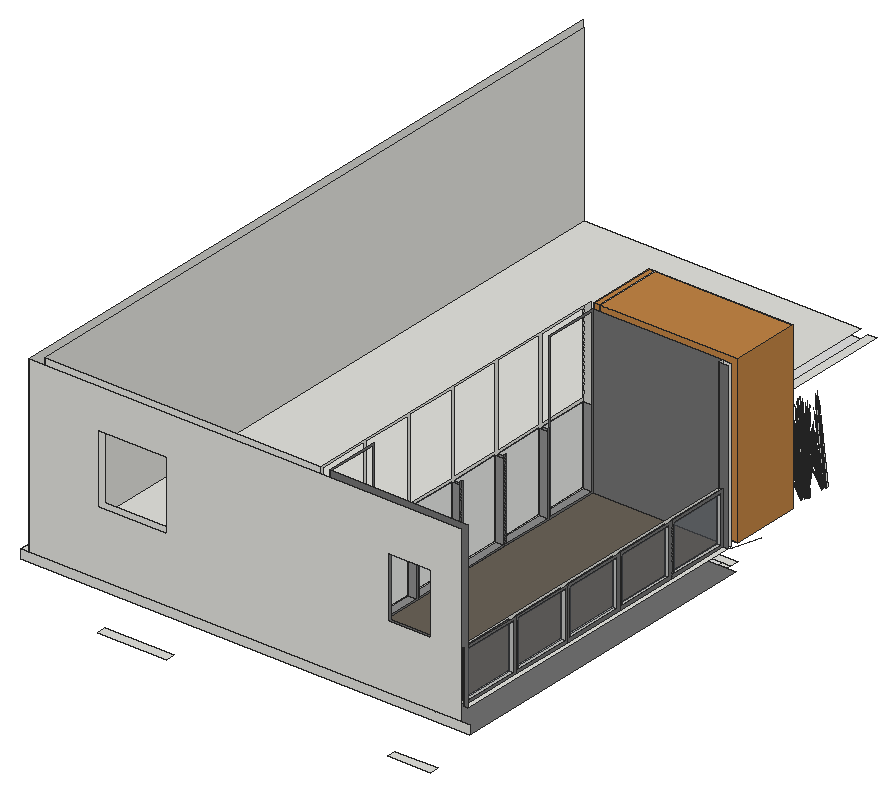
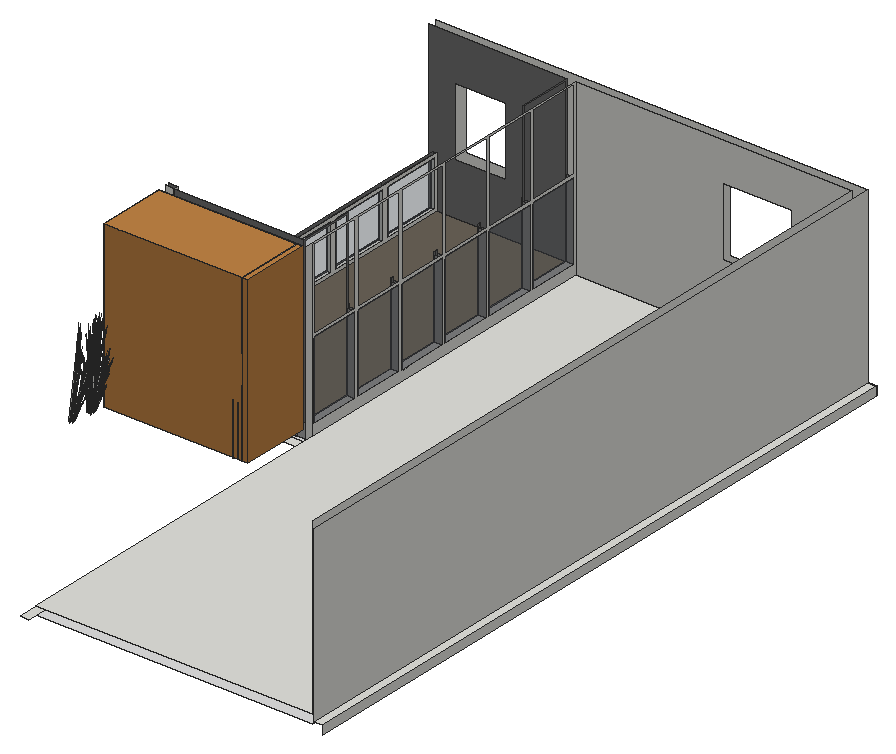
# SketchUp Ruby script. Lengths in inches.
U = 1.inch
M = Sketchup.active_model
def pt(a) = Geom::Point3d.new(a.map { |v| v * U })
def face(e, loops, mat)
  f = e.add_face(loops[0].map { |a| pt(a) })
  loops[1..].each { |l| e.add_face(l.map { |a| pt(a) }).erase! }
  f.material = f.back_material = mat if mat
  f
end
# faces: each face lists its corners as indices into pts; further lists are holes
def faces(e, pts, list, mat = nil) = list.each { |f| face(e, (f[0].is_a?(Array) ? f : [f]).map { |l| l.map { |i| pts[i] } }, mat) }
# xy, xz, yz: faces in a plane at the given z, y or x. An outline is a flat list of corners, or four numbers for a rectangle; further outlines are holes
def ring(l) = l.size == 4 ? [[l[0], l[1]], [l[2], l[1]], [l[2], l[3]], [l[0], l[3]]] : l.each_slice(2).to_a
def flat(e, list, mat, &to3) = list.each { |f| face(e, (f[0].is_a?(Array) ? f : [f]).map { |l| ring(l).map { |u, v| to3.(u, v) } }, mat) }
def xy(e, z, list, mat = nil) = flat(e, list, mat) { |x, y| [x, y, z] }
def xz(e, y, list, mat = nil) = flat(e, list, mat) { |x, z| [x, y, z] }
def yz(e, x, list, mat = nil) = flat(e, list, mat) { |y, z| [x, y, z] }
def lines(e, pts, list) = list.each { |a, b| e.add_line(pt(pts[a]), pt(pts[b])) }
# prism: a flat outline (further loops are holes) pulled along v
def prism(e, loops, v, mat = nil)
  f = face(e, loops, mat); d = Geom::Vector3d.new(v.map { |x| x * U })
  f.pushpull(f.normal.samedirection?(d) ? d.length : -d.length)
end
def box(e, o, s, mat = nil) = prism(e, [[o, [o[0] + s[0], o[1], o[2]], [o[0] + s[0], o[1] + s[1], o[2]], [o[0], o[1] + s[1], o[2]]]], [0, 0, s[2]], mat)
def at(x, y, z, deg = 0) = Geom::Transformation.translation(pt([x, y, z])) * Geom::Transformation.rotation(ORIGIN, Z_AXIS, deg.degrees)
def axes(o, x, y, z) = Geom::Transformation.new([*x, 0, *y, 0, *z, 0, *pt(o).to_a, 1])
def part(name) = M.definitions.add(name)
# library, detail: a bought-in or finely detailed component or shape, given as its bounding box
def library(name, o, s) = part(name).tap { |d| box(d.entities, o, s) }
def detail(e, o, s) = box(e.add_group.entities, o, s)
def put(e, d, t, mat = nil) = e.add_instance(d, t).tap { |i| i.material = mat if mat }
def group(e, t, mat = nil) = e.add_group.tap { |g| g.transformation = t; g.material = mat if mat }.entities
root = M.entities
M.materials.add("Glass_Basic_01").color = [105, 113, 122]
M.materials["Glass_Basic_01"].alpha = 0.25
M.materials.add("LightPink_Translucent").color = [144, 107, 117]
M.materials["LightPink_Translucent"].alpha = 0.75
M.materials.add("M01_Silver_Fog").color = [224, 224, 224]
M.materials.add("M04_Stone_Frost").color = [142, 142, 142]
M.materials.add("M06_Steel_Smoke").color = [114, 114, 114]
M.materials.add("Plaster_04_1K").color = [106, 98, 87]
M.materials.add("Wood_Floor_01_1K").color = [193, 132, 69]
c1 = part("Group\#1")
box(c1.entities,[-3.94,0,0],[99.94,48,114])
c2 = part("blade")
p = [[2.15,0.21,22],[0,0.17,0],[0.09,0.45,0],[2.18,0.31,22],[2.29,0.31,22],[0.38,0.45,0],
  [2.48,0.24,33],[2.49,0.24,33],[2.48,0.22,33]]
faces(c2.entities,p,[[0,1,2,3],[4,5,2,3],[6,3,4,7],[8,0,3,6]])
c3 = part("seeds")
p = [[0.3,-0.1,1.38],[-0.01,-0.03,1.59],[-0.01,-0.03,0.03],[0.14,-0.07,-0.07],[0.29,-0.03,3],[0.15,0.01,3.11]]
faces(c3.entities,p,[[0,1,2,3],[1,0,4,5]],"LightPink_Translucent")
c4 = part("blade with seeds")
put(c4.entities,c2,at(0,0,0))
put(c4.entities,c3,axes([2.4,0.25,30.99],[1.5799,-0.05474,1.17369],[-0.12525,1.92788,0.29478],[-0.07173,-0.02425,1.56792]))
xy(root,477,[[255,0,285,6]])
xy(root,483,[[54,0,102,6]])
xy(root,509,[[204,7,210,43],[204,45,210,81],[204,83,210,119],[204,121,210,157],[204,159,210,195],
  [204,197,210,233]])
xy(root,510,[[0,0,6,231],[6,0,306,0,306,6,210,6,210,231,204,231,204,6,12,6,12,231,6,231],[204,231,210,231,210,234,306,234,306,240,210,240,210,480,204,480],[300,231,306,234]])
xy(root,510,[[12,231,204,474],[210,231,300,234]],"M01_Silver_Fog")
xy(root,510,[[306,0,306,6,210,6,210,231,312,231,312,0],[12,6,204,231]],"M06_Steel_Smoke")
xy(root,516,[[0,0,6,480],[12,6,204,474]])
xy(root,522,[[303,6,306,231]])
xy(root,522,[[210,6,300,234]],"Plaster_04_1K")
xy(root,523,[[204,7,210,43],[204,45,210,81],[204,83,210,119],[204,121,210,157],[204,159,210,195],
  [204,197,210,233]],"M04_Stone_Frost")
xy(root,524,[[300,8,303,49],[300,53,303,94],[300,98,303,139],[300,143,303,184],[300,188,303,229]])
xz(root,0,[[0,510,312,516],[[6,516,306,636],[54,561,102,609],[255,561,285,603]]])
xz(root,6,[[[12,516,204,636],[54,561,102,609]]])
xz(root,6,[[[210,522,210,636,306,636,306,522,303,522,303,558,300,558,300,522],[252,558,288,606]]],"M06_Steel_Smoke")
xz(root,7,[[204,523,210,577]],"M04_Stone_Frost")
xz(root,8,[[300,524,303,556]])
xz(root,43,[[204,523,210,577]],"M04_Stone_Frost")
xz(root,45,[[204,523,210,577]],"M04_Stone_Frost")
xz(root,49,[[300,524,303,556]])
xz(root,53,[[300,524,303,556]])
xz(root,81,[[204,523,210,577]],"M04_Stone_Frost")
xz(root,83,[[204,523,210,577]],"M04_Stone_Frost")
xz(root,94,[[300,524,303,556]])
xz(root,98,[[300,524,303,556]])
xz(root,119,[[204,523,210,577]],"M04_Stone_Frost")
xz(root,121,[[204,523,210,577]],"M04_Stone_Frost")
xz(root,139,[[300,524,303,556]])
xz(root,143,[[300,524,303,556]])
xz(root,157,[[204,523,210,577]],"M04_Stone_Frost")
xz(root,159,[[204,523,210,577]],"M04_Stone_Frost")
xz(root,184,[[300,524,303,556]])
xz(root,188,[[300,524,303,556]])
xz(root,195,[[204,523,210,577]],"M04_Stone_Frost")
xz(root,197,[[204,523,210,577]],"M04_Stone_Frost")
xz(root,229,[[300,524,303,556]])
xz(root,231,[[303,522,306,522,306,636,300,636,300,558,303,558]],"M06_Steel_Smoke")
xz(root,233,[[204,523,210,577]],"M04_Stone_Frost")
xz(root,234,[[300,522,306,636]])
xz(root,234,[[210,522,300,636]],"M06_Steel_Smoke")
xz(root,243,[[213,522,305.51,558]],"M01_Silver_Fog")
xz(root,246,[[216,522,303.26,558]],"M01_Silver_Fog")
xz(root,287.79,[[213,522,216,558]],"M01_Silver_Fog")
yz(root,0,[[0,510,480,516]])
yz(root,6,[[0,516,480,636]])
yz(root,12,[[6,516,474,636]])
yz(root,204,[[[6,516,234,636],[7,579,43,635],[121,579,157,635],[159,579,195,635],[197,579,233,635],[45,579,81,635],[83,579,119,635],[7,523,43,577],[197,523,233,577],[159,523,195,577],[121,523,157,577],[45,523,81,577],[83,523,119,577]],[234,516,240,636]])
yz(root,204,[[7,523,43,577],[45,523,81,577],[83,523,119,577],[121,523,157,577],[159,523,195,577],
  [197,523,233,577]],"Glass_Basic_01")
yz(root,210,[[240,522,288,522,288,568.46,286.46,568.46,286.46,589.54,288,589.54,288,636,240,636]])
yz(root,210,[[6,522,44,522,44,579,43,579,43,523,7,523,7,635,43,635,43,579,44,579,44,636,6,636],[44,522,82,522,82,579,81,579,81,523,45,523,45,579,44,579],[82,522,120,522,120,579,119,579,119,523,83,523,83,579,82,579],[120,522,158,522,158,579,157,579,157,523,121,523,121,579,120,579],[158,522,196,522,196,579,195,579,195,523,159,523,159,579,158,579],
  [196,522,234,522,234,636,196,636,196,579,197,579,197,635,233,635,233,523,197,523,197,579,196,579]],"M06_Steel_Smoke")
yz(root,213,[[243,522,287.79,558]],"M01_Silver_Fog")
yz(root,216,[[246,522,287.79,558]],"M01_Silver_Fog")
yz(root,300,[[[6,522,231,558],[8,524,49,556],[143,524,184,556],[188,524,229,556],[53,524,94,556],[98,524,139,556]],[231,522,234,636]])
yz(root,300,[[8,524,49,556],[53,524,94,556],[98,524,139,556],[143,524,184,556],[188,524,229,556]],"Glass_Basic_01")
yz(root,303,[[8,524,49,556],[53,524,94,556],[98,524,139,556],[143,524,184,556],[188,524,229,556]],"Glass_Basic_01")
yz(root,303,[[[6,522,51,558],[8,524,49,556]],[[51,522,96,558],[53,524,94,556]],[[96,522,141,558],[98,524,139,556]],[[141,522,186,558],[143,524,184,556]],[[186,522,231,558],[188,524,229,556]]],"M06_Steel_Smoke")
p = [[303.26,246,558],[306,255.36,558],[306,255.36,522],[303.26,246,522],[210,240,516],[210,240,522],
  [300,240,516],[306,260.5,516],[209.78,288,636],[209.78,288,522],[305.48,242.91,522],[305.48,242.91,558]]
faces(root,p,[[0,1,2,3]],"M01_Silver_Fog")
lines(root,p,[[4,5],[6,4],[6,7],[8,9],[10,11]])
put(root,c1,at(210,240,522),"Wood_Floor_01_1K")
put(root,c4,axes([304.54,297.61,525.875],[0.20841,-0.0122,1.71376],[-0.13825,0.52864,0.13857],[-0.297,-0.0327,0.73262]))
put(root,c4,axes([304.63,298.54,525.875],[0.17434,-0.11391,1.71376],[0.14677,0.52637,0.13857],[-0.27369,0.11897,0.73262]))
put(root,c4,axes([304.09,299.43,524.59],[0.17462,0.04421,1.43002],[0.11254,0.45156,-0.30754],[-0.23719,0.08453,0.61141]))
put(root,c4,axes([305.63,297.99,525.34],[0.14282,-0.0779,1.77064],[0.04925,0.54394,0.13857],[-0.30935,0.07218,0.63284]))
put(root,c4,axes([305.17,297.11,526.98],[-0.50227,-0.01297,-0.71045],[0.03373,-0.54602,0.08574],[-0.21278,-0.05762,1.00501]))
put(root,c4,axes([304.76,297.25,524.59],[0.0981,0.14994,1.43002],[-0.22605,0.40756,-0.30754],[-0.23211,-0.09741,0.61141]))
put(root,c4,axes([304.36,298.06,526.53],[-0.41757,-0.15024,-0.35414],[0.12179,-0.4383,0.4572],[-0.16812,0.04019,0.87481]))
put(root,c4,axes([304.9375,296.76,525.875],[0.18664,0.09279,1.71376],[-0.38624,0.38925,0.13857],[-0.24072,-0.1756,0.73262]))
put(root,c4,axes([306.06,313.64,525.875],[0.20841,-0.0122,1.71376],[-0.13825,0.52864,0.13857],[-0.297,-0.0327,0.73262]))
put(root,c4,axes([304.65,298.28,526.68],[-0.13612,0.48987,-0.51099],[-0.46669,-0.16791,-0.3958],[-0.1879,0.04492,0.97773]))
put(root,c4,axes([305,297.22,526.68],[-0.36484,0.35674,-0.51099],[-0.31952,-0.37685,-0.3958],[-0.18537,-0.05428,0.97773]))
put(root,c4,axes([304.41,298.25,523.49],[0.01274,0.08487,1.76342],[-0.25688,0.44323,-0.26939],[-0.18246,-0.02234,0.30037]))
put(root,c4,axes([303.72,300.38,524.77],[0.2094,-0.24408,1.1486],[0.08263,0.38639,0.84392],[-0.15132,0.06919,0.25299]))
put(root,c4,axes([304.87,296.89,526.53],[-0.28589,-0.33718,-0.35414],[0.32644,-0.31919,0.4572],[-0.16586,-0.04856,0.87481]))
put(root,c4,axes([305.27,298.89,525.875],[0.1255,-0.16547,1.71376],[0.31687,0.44665,0.13857],[-0.21734,0.2034,0.73262]))
put(root,c4,axes([304.51,299.32,526.53],[-0.43736,0.07697,-0.35414],[-0.11549,-0.43998,0.4572],[-0.12533,0.11818,0.87481]))
put(root,c4,axes([304.27,300.63,523.49],[0.0674,0.0538,1.76342],[0.11428,0.49852,-0.26939],[-0.14937,0.10631,0.30037]))
put(root,c4,axes([304.18,297.7,524.77],[0.32078,-0.03854,1.1486],[-0.20348,0.33954,0.84392],[-0.15852,-0.05093,0.25299]))
put(root,c4,axes([307.14,314.02,525.34],[0.14282,-0.0779,1.77064],[0.04925,0.54394,0.13857],[-0.30935,0.07218,0.63284]))
put(root,c4,axes([306.68,313.15,526.98],[-0.50227,-0.01297,-0.71045],[0.03373,-0.54602,0.08574],[-0.21278,-0.05762,1.00501]))
put(root,c4,axes([306.27,313.28,524.59],[0.0981,0.14994,1.43002],[-0.22605,0.40756,-0.30754],[-0.23211,-0.09741,0.61141]))
put(root,c4,axes([305.17,299.3,525.875],[0.09355,-0.18511,1.71376],[0.39247,0.38307,0.13857],[-0.17705,0.23875,0.73262]))
put(root,c4,axes([305.87,314.09,526.53],[-0.41757,-0.15024,-0.35414],[0.12179,-0.4383,0.4572],[-0.16812,0.04019,0.87481]))
put(root,c4,axes([306.45,312.79,525.875],[0.18664,0.09279,1.71376],[-0.38624,0.38925,0.13857],[-0.24072,-0.1756,0.73262]))
put(root,c4,axes([304.875,299.375,526.68],[0.12908,0.49174,-0.51099],[-0.48882,0.08602,-0.3958],[-0.14008,0.13208,0.97773]))
put(root,c4,axes([306.09,299.02,524.06],[-0.52267,-0.08829,-0.62353],[0.11029,-0.54463,-0.16365],[-0.15598,-0.06599,1.37633]))
put(root,c4,axes([306.51,313.26,526.68],[-0.36484,0.35674,-0.51099],[-0.31952,-0.37685,-0.3958],[-0.18537,-0.05428,0.97773]))
put(root,c4,axes([305.92,314.29,523.49],[0.01274,0.08487,1.76342],[-0.25688,0.44323,-0.26939],[-0.18246,-0.02234,0.30037]))
put(root,c4,axes([306.04,296.47,526.98],[-0.42844,-0.2603,-0.71045],[0.30448,-0.45614,0.08574],[-0.15523,-0.15542,1.00501]))
put(root,c4,axes([305.84,296.48,526.68],[-0.4958,0.12802,-0.51099],[-0.08673,-0.48481,-0.3958],[-0.13317,-0.13893,0.97773]))
put(root,c4,axes([305.41,300.05,524.02],[-0.47024,-0.26927,-0.49651],[0.28107,-0.48284,0],[-0.1071,-0.06133,1.57504]))
put(root,c4,axes([305.2,296.04,523.49],[-0.04867,0.07094,1.76342],[-0.49185,0.15296,-0.26939],[-0.11882,-0.13915,0.30037]))
put(root,c4,axes([305.69,300.38,524.375],[-0.31414,0.53965,0],[-0.52557,-0.30095,-0.51607],[-0.1197,-0.06854,1.63711]))
put(root,c4,axes([306.375,312.92,526.53],[-0.28589,-0.33718,-0.35414],[0.32644,-0.31919,0.4572],[-0.16586,-0.04856,0.87481]))
put(root,c4,axes([305.69,313.73,524.77],[0.32078,-0.03854,1.1486],[-0.20348,0.33954,0.84392],[-0.15852,-0.05093,0.25299]))
put(root,c4,axes([305.12,301.16,524.59],[0.15856,-0.08496,1.43002],[0.39147,0.25616,-0.30754],[-0.11652,0.22165,0.61141]))
put(root,c4,axes([304.89,296.31,524.13],[-0.14494,0.43975,-0.03893],[-0.4461,-0.13527,-0.17649],[-0.06773,-0.07192,0.58215]))
put(root,c4,axes([305.5625,295.76,524.59],[-0.03043,0.17617,1.43002],[-0.4448,0.14748,-0.30754],[-0.10397,-0.22771,0.61141]))
put(root,c4,axes([305.71,296.22,525.875],[0.11485,0.17291,1.71376],[-0.53072,0.14557,0.13857],[-0.11995,-0.27145,0.73262]))
put(root,c4,axes([306.6875,299.1,524.67],[-0.5073,0.35754,-0.29095],[-0.33735,-0.5052,-0.50002],[-0.12516,-0.05131,1.59708]))
put(root,c4,axes([305.89,296.125,526.53],[-0.0776,-0.43378,-0.35414],[0.44361,-0.11454,0.4572],[-0.11915,-0.12431,0.87481]))
put(root,c4,axes([304.66,298.32,524.375],[-0.62828,0,0],[0,-0.6019,-0.51607],[0,-0.13709,1.63711]))
put(root,c4,axes([305.54,299.85,524.03],[-0.11803,-0.46926,-0.30978],[0.46876,-0.13325,0.30978],[-0.0945,-0.05411,1.38974]))
put(root,c4,axes([305.28,300.34,526.53],[-0.33997,0.28354,-0.35414],[-0.32182,-0.32376,0.4572],[-0.04897,0.1645,0.87481]))
put(root,c4,axes([307.02,299.49,524.06],[-0.33843,0.40479,-0.62353],[-0.42041,-0.36705,-0.16365],[-0.13561,0.10098,1.37633]))
put(root,c4,axes([307.6,315.06,524.06],[-0.52267,-0.08829,-0.62353],[0.11029,-0.54463,-0.16365],[-0.15598,-0.06599,1.37633]))
put(root,c4,axes([305.14,298.16,524.33],[-0.46736,0.45277,0.30756],[-0.46764,-0.44801,-0.36492],[-0.01632,-0.12858,1.64885]))
put(root,c4,axes([307.07,299.42,525.33],[0.4342,0.21716,1.51261],[-0.42537,0.46784,0.59816],[-0.19053,-0.27728,1.26806]))
put(root,c4,axes([307.55,312.5,526.98],[-0.42844,-0.2603,-0.71045],[0.30448,-0.45614,0.08574],[-0.15523,-0.15542,1.00501]))
put(root,c4,axes([307.35,312.52,526.68],[-0.4958,0.12802,-0.51099],[-0.08673,-0.48481,-0.3958],[-0.13317,-0.13893,0.97773]))
put(root,c4,axes([305.41,295.48,524.77],[0.2621,0.18744,1.1486],[-0.38171,0.11267,0.84392],[-0.08167,-0.14405,0.25299]))
put(root,c4,axes([307.26,299.27,524.46],[-0.49063,-0.43346,-0.25192],[0.41285,-0.48673,0.5513],[-0.13212,0.05071,1.68216]))
put(root,c4,axes([306.36,298.85,524.21],[-0.30184,-0.45202,-0.44739],[0.45719,-0.31831,0.21531],[-0.09768,-0.05593,1.43643]))
put(root,c4,axes([305.51,300.04,527.34],[-0.01307,0.49815,-0.7886],[-0.55054,-0.03346,0.09517],[-0.0581,0.21104,1.11556]))
put(root,c4,axes([306.92,316.09,524.02],[-0.47024,-0.26927,-0.49651],[0.28107,-0.48284,0],[-0.1071,-0.06133,1.57504]))
put(root,c4,axes([306.71,312.08,523.49],[-0.04867,0.07094,1.76342],[-0.49185,0.15296,-0.26939],[-0.11882,-0.13915,0.30037]))
put(root,c4,axes([305.5,301.44,524.77],[-0.013,-0.32022,1.1486],[0.32493,0.22839,0.84392],[-0.0639,0.15263,0.25299]))
put(root,c4,axes([307.01,299.17,524.21],[-0.54562,0.03324,-0.44739],[-0.04934,-0.55185,0.21531],[-0.09768,0.05593,1.43643]))
put(root,c4,axes([305.96,300.1,524.48],[0.47024,0.26927,0.49651],[-0.28107,0.48284,0],[-0.1071,-0.06133,1.57504]))
put(root,c4,axes([305.32,300.74,525.36],[0.01104,-0.27801,1.54345],[0.49652,0.14685,0.21329],[-0.04302,0.2963,0.72882]))
put(root,c4,axes([306.41,299.11,524.4375],[0.13317,-0.63814,-0.23429],[0.63143,0.11124,0.51271],[-0.11033,-0.08813,1.5644]))
put(root,c4,axes([306.64,299.26,524.62],[-0.09693,0.48062,0.1448],[-0.47357,-0.08343,-0.41347],[-0.08619,-0.04935,1.26744]))
put(root,c4,axes([306.41,312.35,524.13],[-0.14494,0.43975,-0.03893],[-0.4461,-0.13527,-0.17649],[-0.06773,-0.07192,0.58215]))
put(root,c4,axes([307.58,300.6,524.02],[-0.47024,0.26927,-0.49651],[-0.28107,-0.48284,0],[-0.1071,0.06133,1.57504]))
put(root,c4,axes([304.8,297.91,524.02],[0,-0.53854,-0.49651],[0.56215,0,0],[0,-0.12266,1.57504]))
put(root,c4,axes([305.04,298.41,524.48],[0,0.53854,0.49651],[-0.56215,0,0],[0,-0.12266,1.57504]))
put(root,c4,axes([307.61,300.45,524.19],[-0.31023,-0.54153,-0.05142],[0.52557,-0.30095,0.51607],[-0.12951,0.05156,1.6363]))
put(root,c4,axes([307.07,311.79,524.59],[-0.03043,0.17617,1.43002],[-0.4448,0.14748,-0.30754],[-0.10397,-0.22771,0.61141]))
put(root,c4,axes([305.62,300.21,527],[0.35968,0.36185,-0.5672],[-0.37996,0.3169,-0.43934],[-0.05473,0.18385,1.08528]))
put(root,c4,axes([307.22,312.25,525.875],[0.11485,0.17291,1.71376],[-0.53072,0.14557,0.13857],[-0.11995,-0.27145,0.73262]))
put(root,c4,axes([307.47,300.38,524.03],[-0.46876,-0.13325,-0.30978],[0.11803,-0.46926,0.30978],[-0.0945,0.05411,1.38974]))
put(root,c4,axes([308.2,315.14,524.67],[-0.5073,0.35754,-0.29095],[-0.33735,-0.5052,-0.50002],[-0.12516,-0.05131,1.59708]))
put(root,c4,axes([306.26,298.54,524.67],[-0.56585,-0.25696,-0.29095],[0.27246,-0.54236,-0.50002],[-0.01778,-0.13316,1.59708]))
put(root,c4,axes([307.74,298.38,524.84],[-0.01373,-0.50706,1.41272],[0.62119,0.13144,0.59816],[-0.14692,0.27746,1.3335]))
put(root,c4,axes([307.4,312.16,526.53],[-0.0776,-0.43378,-0.35414],[0.44361,-0.11454,0.4572],[-0.11915,-0.12431,0.87481]))
put(root,c4,axes([306.17,314.36,524.375],[-0.62828,0,0],[0,-0.6019,-0.51607],[0,-0.13709,1.63711]))
put(root,c4,axes([307.05,315.89,524.03],[-0.11803,-0.46926,-0.30978],[0.46876,-0.13325,0.30978],[-0.0945,-0.05411,1.38974]))
put(root,c4,axes([305.23,300.75,524.82],[0.45645,-0.09537,0.06507],[0.10494,0.38421,-0.86304],[-0.02894,0.19449,0.7736]))
put(root,c4,axes([307.39,299.02,524.67],[0.05855,0.61451,-0.29095],[-0.60981,0.03716,-0.50002],[-0.10738,0.08185,1.59708]))
put(root,c4,axes([306.01,297.99,524.1],[-0.20635,-0.55225,-0.69835],[0.59439,-0.19889,-0.18329],[-0.02281,-0.18701,1.54149]))
put(root,c4,axes([306.94,296.26,526.68],[-0.49392,-0.135,-0.51099],[0.1693,-0.46287,-0.3958],[-0.04529,-0.18636,0.97773]))
put(root,c4,axes([306.03,299.6875,525.875],[-0.0123,-0.2067,1.71376],[0.53301,0.13712,0.13857],[-0.03297,0.29456,0.73262]))
put(root,c4,axes([306.65,314.2,524.33],[-0.46736,0.45277,0.30756],[-0.46764,-0.44801,-0.36492],[-0.01632,-0.12858,1.64885]))
